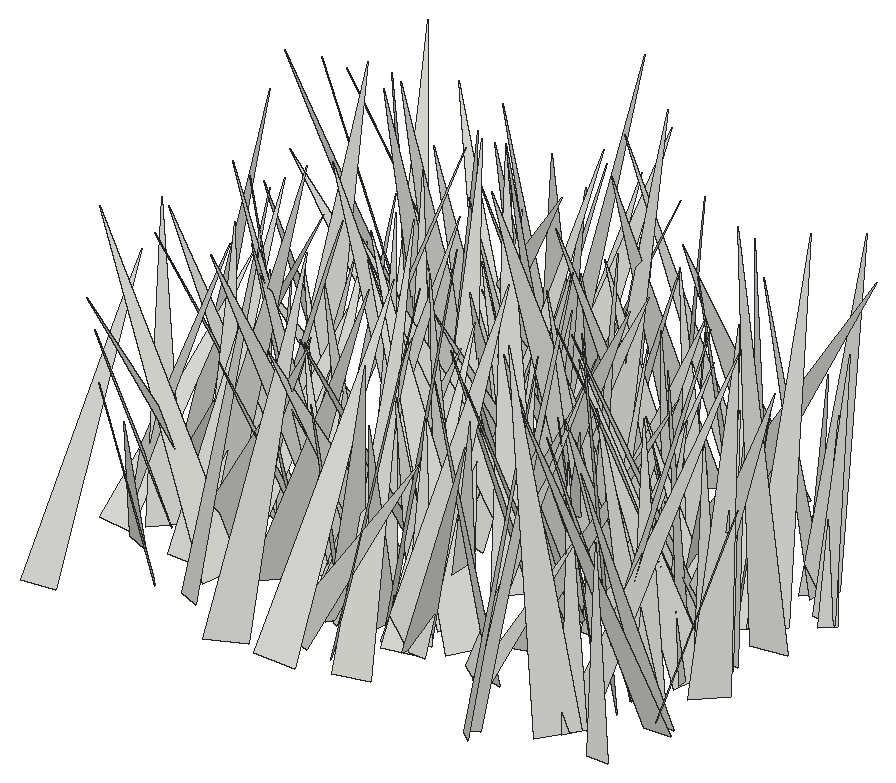
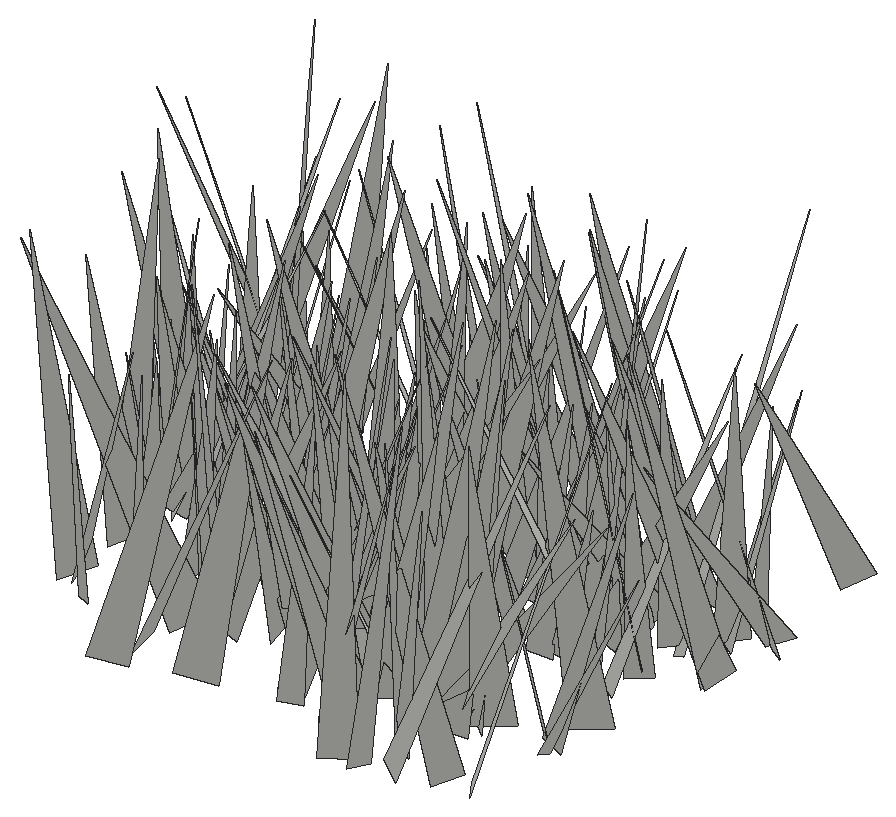
# SketchUp Ruby script. Lengths in inches.
U = 1.inch
M = Sketchup.active_model
def pt(a) = Geom::Point3d.new(a.map { |v| v * U })
def face(e, loops, mat)
  f = e.add_face(loops[0].map { |a| pt(a) })
  loops[1..].each { |l| e.add_face(l.map { |a| pt(a) }).erase! }
  f.material = f.back_material = mat if mat
  f
end
# faces: each face lists its corners as indices into pts; further lists are holes
def faces(e, pts, list, mat = nil) = list.each { |f| face(e, (f[0].is_a?(Array) ? f : [f]).map { |l| l.map { |i| pts[i] } }, mat) }
# xy, xz, yz: faces in a plane at the given z, y or x. An outline is a flat list of corners, or four numbers for a rectangle; further outlines are holes
def ring(l) = l.size == 4 ? [[l[0], l[1]], [l[2], l[1]], [l[2], l[3]], [l[0], l[3]]] : l.each_slice(2).to_a
def flat(e, list, mat, &to3) = list.each { |f| face(e, (f[0].is_a?(Array) ? f : [f]).map { |l| ring(l).map { |u, v| to3.(u, v) } }, mat) }
def xy(e, z, list, mat = nil) = flat(e, list, mat) { |x, y| [x, y, z] }
def xz(e, y, list, mat = nil) = flat(e, list, mat) { |x, z| [x, y, z] }
def yz(e, x, list, mat = nil) = flat(e, list, mat) { |y, z| [x, y, z] }
def lines(e, pts, list) = list.each { |a, b| e.add_line(pt(pts[a]), pt(pts[b])) }
# prism: a flat outline (further loops are holes) pulled along v
def prism(e, loops, v, mat = nil)
  f = face(e, loops, mat); d = Geom::Vector3d.new(v.map { |x| x * U })
  f.pushpull(f.normal.samedirection?(d) ? d.length : -d.length)
end
def box(e, o, s, mat = nil) = prism(e, [[o, [o[0] + s[0], o[1], o[2]], [o[0] + s[0], o[1] + s[1], o[2]], [o[0], o[1] + s[1], o[2]]]], [0, 0, s[2]], mat)
def at(x, y, z, deg = 0) = Geom::Transformation.translation(pt([x, y, z])) * Geom::Transformation.rotation(ORIGIN, Z_AXIS, deg.degrees)
def axes(o, x, y, z) = Geom::Transformation.new([*x, 0, *y, 0, *z, 0, *pt(o).to_a, 1])
def part(name) = M.definitions.add(name)
# library, detail: a bought-in or finely detailed component or shape, given as its bounding box
def library(name, o, s) = part(name).tap { |d| box(d.entities, o, s) }
def detail(e, o, s) = box(e.add_group.entities, o, s)
def put(e, d, t, mat = nil) = e.add_instance(d, t).tap { |i| i.material = mat if mat }
def group(e, t, mat = nil) = e.add_group.tap { |g| g.transformation = t; g.material = mat if mat }.entities
root = M.entities
c1 = part("fur_instance\#9")
p = [[0.8125,0,1.79],[0.67,-0.02,1.48],[0,-0.11,0],[0,0.11,0]]
faces(c1.entities,p,[[0,1,2,3]])
put(root,c1,axes([138.79,216.625,-27.1],[-2.84095,-2.72325,0.75235],[-2.80656,2.8428,-0.30791],[0.32453,0.74533,3.9233]))
put(root,c1,axes([145.17,216.32,-27.1],[2.54302,-4.52945,1.06711],[-4.23804,-1.75205,2.66287],[1.92189,2.12978,4.46004]))
put(root,c1,axes([158.66,216.3125,-27.1],[-0.06677,3.94377,1.582],[4.24655,0.00562,0.16522],[-0.15123,-1.5834,3.94087]))
put(root,c1,axes([143.4,214.84,-27.1],[5.43285,-3.6045,3.64876],[-4.74936,-5.54221,1.59663],[-1.93634,3.48041,6.32132]))
put(root,c1,axes([156.51,216.85,-27.1],[-5.45216,4.70878,2.71596],[5.23215,5.58914,0.81316],[1.47433,-2.42158,7.15803]))
put(root,c1,axes([136.69,218.34,-27.1],[-0.43336,-3.79274,0.22877],[-3.61563,0.48241,1.14868],[1.16807,0.08612,3.64049]))
put(root,c1,axes([135.86,213.875,-27.1],[-4.59878,4.14257,0.47856],[3.69105,4.37512,-2.40275],[1.94062,1.49539,5.70408]))
put(root,c1,axes([146.57,216.95,-27.1],[7.04246,3.4796,1.7186],[3.70112,-7.09298,-0.80545],[-1.16744,-1.49647,7.81378]))
put(root,c1,axes([154.09,214.77,-27.1],[4.5947,4.98178,1.41698],[4.55399,-4.78808,2.06705],[-2.46722,0.43974,6.4542]))
put(root,c1,axes([137.43,221.86,-27.1],[-5.00279,-6.48805,0.18943],[-5.66686,4.48249,3.86684],[3.16501,-2.22958,7.22289]))
put(root,c1,axes([145.65,218.68,-27.1],[5.23742,-3.794,0.7561],[-3.79638,-5.28528,-0.22367],[-0.74406,0.26094,6.46336]))
put(root,c1,axes([145.58,214.8,-27.1],[-1.59566,7.05244,0.57454],[6.94745,1.67322,-1.24356],[1.34162,-0.27674,7.12297]))
put(root,c1,axes([159.07,219.14,-27.1],[-1.75901,-6.72397,0.92553],[-6.70142,1.56883,-1.33876],[-1.07676,1.22044,6.82009]))
put(root,c1,axes([148.83,218.63,-27.1],[5.31861,-1.95589,0.12332],[-1.94358,-5.30997,-0.39374],[-0.25139,-0.32717,5.65315]))
put(root,c1,axes([146.96,219.07,-27.1],[4.83805,-1.95602,0.87332],[-1.75837,-4.85831,-1.14034],[-1.22345,-0.75248,5.09238]))
put(root,c1,axes([152.3,217.64,-27.1],[2.38056,3.51502,0.37387],[3.33138,-2.08023,-1.65431],[1.18197,-1.21634,3.90969]))
put(root,c1,axes([138.8,219.61,-27.1],[2.77166,-6.45652,0.14972],[-5.9267,-2.47813,2.8503],[2.56578,1.25036,6.42219]))
put(root,c1,axes([156.83,217.34,-27.1],[-4.5869,1.43943,1.05541],[1.33614,4.69877,-0.60151],[1.18347,0.27406,4.76967]))
put(root,c1,axes([144.97,219.27,-27.1],[3.60771,1.96245,2.32029],[2.67745,-3.75626,-0.98607],[-1.43745,-2.07119,3.98679]))
put(root,c1,axes([158.9,219.59,-27.1],[-0.82643,-5.48525,0.94931],[-5.54864,0.73423,-0.58792],[-0.44918,1.02229,5.51591]))
put(root,c1,axes([140.375,218.38,-27.1],[-6.66331,2.16551,0.21128],[2.17487,6.60915,0.85019],[-0.06344,-0.87375,6.95459]))
put(root,c1,axes([156.39,220.07,-27.1],[-5.2101,-5.93708,2.74108],[-5.84341,5.80017,1.45611],[2.93548,1.00834,7.76362]))
put(root,c1,axes([136.41,220.42,-27.1],[-3.04266,-3.74721,0.50143],[-3.60797,3.07034,1.05183],[1.12942,-0.28668,4.71094]))
put(root,c1,axes([142.25,221.5,-27.1],[-3.9218,-4.42687,0.35438],[-4.07666,3.77609,2.05553],[1.7617,-1.11678,5.54549]))
put(root,c1,axes([148.41,215.53,-27.1],[0.0768,8.17284,0.16546],[8.06568,-0.10268,1.32775],[-1.3295,-0.15078,8.06464]))
put(root,c1,axes([141.87,219.17,-27.1],[6.48225,-3.39085,0.68777],[-3.4557,-6.41712,0.9323],[-0.17042,1.14593,7.25591]))
put(root,c1,axes([152.53,218.3,-27.1],[-3.42492,-4.02626,1.68032],[-4.34426,2.9504,-1.78518],[-0.40205,2.41841,4.97534]))
put(root,c1,axes([148.8,218.72,-27.1],[-2.37433,3.47563,1.70417],[3.72029,2.6012,-0.12184],[1.06942,-1.33243,4.20745]))
put(root,c1,axes([140.53,216.38,-27.1],[3.83849,6.3713,1.10198],[6.13828,-3.99344,1.70758],[-2.03209,-0.02789,7.23959]))
put(root,c1,axes([144.49,219.02,-27.1],[1.01992,4.1189,1.46608],[4.23417,-0.55549,-1.38501],[1.0893,-1.69737,4.0109]))
put(root,c1,axes([144.74,222.35,-27.1],[-6.04066,-0.63869,2.51357],[0.73038,5.69455,3.20222],[2.48847,-3.22176,5.16172]))
put(root,c1,axes([156.6,220.88,-27.1],[-4.48519,-3.52054,0.94744],[-3.42145,4.58335,0.83384],[1.25916,-0.08621,5.64055]))
put(root,c1,axes([148.57,218.1875,-27.1],[-1.59502,6.99566,2.35908],[7.02793,2.17795,-1.70682],[2.26111,-1.83463,6.96922]))
put(root,c1,axes([146.97,219.4,-27.1],[7.03431,3.48518,2.0857],[3.73576,-7.18871,-0.58711],[-1.59396,-1.46769,7.82836]))
put(root,c1,axes([148.51,221.25,-27.1],[-2.23247,-5.83337,0.18602],[-5.6892,2.13065,-1.46288],[-1.30221,0.692,6.07224]))
put(root,c1,axes([154.09,215.2,-27.1],[4.35175,7.0169,0.44581],[6.16578,-4.0605,3.72408],[-3.37917,1.6275,7.36925]))
put(root,c1,axes([149.11,220.74,-27.1],[4.27597,-2.96302,0.67606],[-2.94629,-4.32773,-0.33261],[-0.74558,0.10858,5.19161]))
put(root,c1,axes([142.72,220.2,-27.1],[-2.07432,-2.92088,0.84042],[-3.01146,2.11274,-0.09003],[0.41107,0.73854,3.58137]))
put(root,c1,axes([147.82,220.33,-27.1],[-3.6167,2.28369,2.19841],[2.80718,3.85669,0.61192],[1.47241,-1.74341,4.23336]))
put(root,c1,axes([144.92,220.76,-27.1],[1.50784,-3.41822,0.5063],[-3.4457,-1.52893,-0.06057],[-0.26023,0.4385,3.73552]))
put(root,c1,axes([143.4,222.04,-27.1],[1.95168,-6.84621,1.26966],[-6.52036,-2.2596,-2.16121],[-2.44285,0.56154,6.78298]))
put(root,c1,axes([144.15,220.08,-27.1],[4.85202,-3.37562,1.03104],[-3.52041,-4.75453,1.00059],[-0.25408,1.41409,5.82544]))
put(root,c1,axes([156.39,218.14,-27.1],[3.64323,6.95762,0.66244],[6.95502,-3.53547,-1.11744],[0.68929,-1.10109,7.77386]))
put(root,c1,axes([158.26,220.34,-27.1],[4.88732,1.92922,0.49219],[1.99044,-4.76555,-1.08522],[-0.04774,-1.19066,5.14102]))
put(root,c1,axes([134.9,219.64,-27.1],[4.20289,4.66758,0.96744],[4.74909,-3.98911,-1.38552],[0.41036,-1.63927,6.12625]))
put(root,c1,axes([150.39,219.59,-27.1],[-4.97351,5.86998,1.15657],[5.9442,4.67754,1.82131],[-0.6788,-2.04794,7.47498]))
put(root,c1,axes([153.36,221.65,-27.1],[-2.96525,-5.05492,0.58848],[-5.08807,2.93137,-0.45808],[-0.10025,0.73898,5.84252]))
put(root,c1,axes([144.8,218.58,-27.1],[3.51205,7.24819,1.1392],[7.33442,-3.43356,-0.76524],[0.20101,-1.35755,8.01781]))
put(root,c1,axes([156.36,218.76,-27.1],[5.62974,5.25868,1.12192],[5.27805,-5.71471,0.30107],[-1.02693,-0.54292,7.69786]))
put(root,c1,axes([144.77,219.97,-27.1],[-7.94923,-1.56442,0.5472],[-1.62855,7.87073,-1.15603],[0.30767,1.24144,8.0188]))
put(root,c1,axes([157.41,220.55,-27.1],[0.3865,-5.10308,2.42648],[-5.49086,-0.91339,-1.04632],[-1.33405,2.28099,5.00959]))
put(root,c1,axes([151.42,218.34,-27.1],[3.77289,4.9439,0.17652],[4.9129,-3.7705,0.5956],[-0.58026,0.22179,6.19049]))
put(root,c1,axes([139.36,220.99,-27.1],[3.2608,1.42212,0.87051],[1.60342,-3.19897,-0.78016],[-0.45742,-1.07574,3.47082]))
put(root,c1,axes([136.67,219.89,-27.1],[-4.60516,3.74944,1.60687],[3.84875,4.79672,-0.16237],[1.35183,-0.88372,5.93628]))
put(root,c1,axes([140.39,219.43,-27.1],[4.26964,0.47793,1.18834],[0.14194,-4.28676,1.21405],[-1.27296,1.12502,4.1212]))
put(root,c1,axes([138.6,219.76,-27.1],[7.3545,-2.24014,2.18394],[-2.66673,-7.40612,1.38362],[-1.63595,2.00191,7.56257]))
put(root,c1,axes([157.34,220.75,-27.1],[2.70237,-4.42657,2.31196],[-4.83243,-2.98105,-0.05917],[-1.25989,1.93941,5.18593]))
put(root,c1,axes([148.54,218,-27.1],[-4.13598,4.27474,0.09369],[4.07434,3.97972,-1.71759],[1.29691,1.13001,5.6947]))
put(root,c1,axes([148.81,220.54,-27.1],[-1.16984,-6.03511,2.92768],[-6.70455,0.96018,-0.69968],[-0.2073,3.00298,6.1075]))
put(root,c1,axes([144.25,220.6,-27.1],[2.31719,-2.3997,1.71249],[-2.74416,-2.55172,0.13746],[-1.07739,1.33819,3.33302]))
put(root,c1,axes([151.54,223.72,-27.1],[6.17469,-3.94346,0.96595],[-3.5616,-6.10514,-2.15707],[-1.94909,-1.33681,7.00177]))
put(root,c1,axes([149.03,220.72,-27.1],[-5.22041,4.31379,0.87725],[4.39805,5.05275,1.32586],[-0.18846,-1.57859,6.64105]))
put(root,c1,axes([143.22,220.8,-27.1],[-3.14224,2.77876,1.0294],[2.91205,3.17344,0.32264],[0.54877,-0.92877,4.18224]))
put(root,c1,axes([138.76,218.4,-27.1],[0.11708,7.08162,0.20269],[7.08451,-0.11681,-0.01106],[0.00771,-0.20285,7.08258]))
put(root,c1,axes([154.96,220.86,-27.1],[-3.71707,-2.68533,1.32909],[-2.9797,3.53518,-1.19076],[0.31439,1.75658,4.42828]))
put(root,c1,axes([146.03,220.1,-27.1],[0.42916,7.00561,1.64499],[7.11073,-0.66598,0.98114],[-1.10544,-1.56418,6.94983]))
put(root,c1,axes([157.76,222.74,-27.1],[-5.95975,2.47486,1.75961],[2.91321,5.75356,1.77469],[0.85695,-2.34763,6.20435]))
put(root,c1,axes([156.88,224.47,-27.1],[-5.73536,-5.62008,0.65862],[-5.46135,5.74328,1.44982],[1.48081,-0.58562,7.89796]))
put(root,c1,axes([135.26,218.88,-27.1],[-2.44099,4.81015,0.04297],[4.37742,2.2412,-2.21652],[1.99437,0.96814,4.91762]))
put(root,c1,axes([151.91,223.63,-27.1],[-0.76321,-4.71965,0.1503],[-4.6984,0.77422,0.45372],[0.47201,0.07524,4.75939]))
put(root,c1,axes([140.65,223.77,-27.1],[-0.18064,-6.52008,0.8881],[-6.57997,0.17015,-0.08916],[-0.06535,0.89016,6.52198]))
put(root,c1,axes([137.96,221.34,-27.1],[3.60386,-3.42869,2.87422],[-4.08632,-4.02533,0.32181],[-1.82182,2.24626,4.96388]))
put(root,c1,axes([151.09,224.28,-27.1],[-0.50575,-5.47671,0.42869],[-5.44927,0.55465,0.65709],[0.69543,0.36321,5.46062]))
put(root,c1,axes([138.57,225.09,-27.1],[-4.91582,-6.36103,2.07601],[-5.8042,5.33544,2.60426],[3.32923,-0.09063,7.60565]))
put(root,c1,axes([137.95,223.26,-27.1],[5.79589,4.16761,1.50359],[4.42839,-5.37215,-2.17978],[0.13803,-2.64446,6.79779]))
put(root,c1,axes([137.8125,225.34,-27.1],[-3.98509,-5.15803,0.00595],[-5.07141,3.91953,1.18509],[0.94137,-0.71992,6.40951]))
put(root,c1,axes([151.54,220.64,-27.1],[5.52796,-0.81869,0.7417],[-1.07099,-4.89962,2.57397],[-0.27083,2.66498,4.96017]))
put(root,c1,axes([140.28,222.67,-27.1],[-1.81659,5.58818,1.87966],[5.39696,0.78429,2.88421],[-2.37355,-2.49359,5.11948]))
put(root,c1,axes([158.39,222.79,-27.1],[-3.98978,2.11987,2.03955],[2.3526,4.36264,0.06771],[1.76604,-1.02247,4.51748]))
put(root,c1,axes([139.4,222.57,-27.1],[1.95895,3.98258,1.69888],[4.26762,-2.09086,-0.01944],[-0.73116,-1.53362,4.43825]))
put(root,c1,axes([135.21,222.33,-27.1],[6.85637,-0.90607,0.05149],[-0.90407,-6.7849,0.99057],[0.07926,0.98874,6.84468]))
put(root,c1,axes([149.9,223.8,-27.1],[-2.91722,-4.26379,0.81225],[-4.33997,2.88016,-0.46811],[0.06569,0.93518,5.14499]))
put(root,c1,axes([158.99,222.14,-27.1],[5.64429,-3.09602,3.33103],[-3.78051,-6.14532,0.69416],[-2.52761,2.27789,6.40012]))
put(root,c1,axes([158.16,223.8125,-27.1],[2.54214,-2.62214,0.84113],[-2.70032,-2.59808,0.06187],[-0.53981,0.64801,3.65161]))
put(root,c1,axes([139.62,220.21,-27.1],[-3.68567,4.23937,0.30212],[3.60627,3.33103,-2.74713],[2.24908,1.60613,4.89997]))
put(root,c1,axes([157.61,224.69,-27.1],[-5.40162,-4.18627,0.13743],[-4.18531,5.38577,-0.4449],[-0.16419,0.43574,6.81941]))
put(root,c1,axes([152.88,225.24,-27.1],[2.25117,-4.50739,0.41367],[-4.42833,-2.28883,-0.84056],[-0.93676,-0.01195,4.96767]))
put(root,c1,axes([137.53,223.91,-27.1],[-2.45808,3.26284,2.53045],[3.74921,2.99751,-0.22312],[1.72995,-1.86016,4.07903]))
put(root,c1,axes([157.625,222.51,-27.1],[-5.30333,-1.20318,1.41609],[-1.56427,5.2022,-1.4382],[1.00301,1.75149,5.24448]))
put(root,c1,axes([141.08,221.875,-27.1],[-2.87102,4.68172,0.40163],[4.57171,2.89185,-1.02921],[1.08596,0.20316,5.39463]))
put(root,c1,axes([142.53,224.25,-27.1],[1.52627,-4.48364,1.33128],[-4.39877,-0.90019,2.01128],[1.58937,1.81423,4.28804]))
put(root,c1,axes([156.03,224.47,-27.1],[3.29636,-5.4576,1.30622],[-5.51274,-2.86598,1.93739],[1.04942,2.08768,6.07437]))
put(root,c1,axes([141.25,224.82,-27.1],[0.46643,-4.66615,1.44002],[-4.86096,-0.58186,-0.31092],[-0.46655,1.39737,4.67909]))
put(root,c1,axes([135.65,222.11,-27.1],[-6.79191,0.51616,3.38033],[-0.49773,7.28774,-2.11287],[3.3831,2.10844,6.47551]))
put(root,c1,axes([144.375,225.44,-27.1],[4.0303,-5.81988,3.12764],[-5.66664,-4.92868,-1.86917],[-3.39741,1.31665,6.82792]))
put(root,c1,axes([157.97,223.84,-27.1],[-2.87037,3.7349,1.34525],[3.80013,3.06525,-0.40189],[1.14815,-0.80807,4.69329]))
put(root,c1,axes([149.66,226.02,-27.1],[4.03439,-1.67825,0.01541],[-1.64329,-3.95818,-0.85174],[-0.3411,-0.78061,4.28572]))
put(root,c1,axes([154.6,226.28,-27.1],[4.66467,-0.77947,0.02704],[-0.7406,-4.47818,-1.32848],[-0.24456,-1.30606,4.53893]))
put(root,c1,axes([149.18,223.625,-27.1],[-6.71454,4.39928,1.56364],[4.39375,6.8803,-0.4901],[1.57912,-0.43767,8.0124]))
put(root,c1,axes([154.5625,224.64,-27.1],[0.69151,3.97199,1.28395],[4.17346,-0.6309,-0.296],[0.08642,-1.31479,4.02085]))
put(root,c1,axes([157.38,224.82,-27.1],[-1.85647,3.95367,0.8299],[3.82368,1.42492,1.76516],[-1.30372,-1.4508,3.99527]))
put(root,c1,axes([152.96,223.03,-27.1],[2.80201,6.02167,1.40008],[5.6342,-3.12002,2.14317],[-2.54489,-0.27744,6.28638]))
put(root,c1,axes([147.13,226.45,-27.1],[3.33833,-6.51025,0.54896],[-6.14625,-2.92038,2.74304],[2.21549,1.70799,6.78259]))
put(root,c1,axes([152.72,224.22,-27.1],[2.02103,5.13059,0.73898],[5.12624,-1.86067,-1.10143],[0.76856,-1.08099,5.40318]))
put(root,c1,axes([147.71,226.36,-27.1],[-4.43221,4.72995,1.58971],[4.78005,3.41433,3.16821],[-1.43205,-3.24253,5.65503]))
put(root,c1,axes([158.14,224.45,-27.1],[1.43677,3.63281,1.03111],[3.57622,-1.66329,0.8769],[-1.21291,-0.60083,3.80693]))
put(root,c1,axes([151.29,225.66,-27.1],[-5.71627,0.02456,1.51927],[0.09668,5.9079,0.26822],[1.51639,-0.28405,5.71003]))
put(root,c1,axes([140.52,224.46,-27.1],[-1.14245,4.14217,0.46464],[4.01441,0.96381,1.27839],[-1.12161,-0.76952,4.10226]))
put(root,c1,axes([140.23,223.15,-27.1],[5.64336,5.1887,0.30355],[5.15395,-5.64438,0.66329],[-0.67191,0.28398,7.63742]))
put(root,c1,axes([148.5625,226.45,-27.1],[-1.63509,-3.83691,0.93062],[-3.94815,1.58786,-0.39017],[-0.00453,1.00909,4.15248]))
put(root,c1,axes([145.66,227.8,-27.1],[-0.82646,-4.24361,0.01629],[-4.06802,0.79698,1.2278],[1.20816,-0.21938,4.14533]))
put(root,c1,axes([148.79,224.56,-27.1],[-4.40287,4.25609,0.42122],[4.26988,4.40886,0.08361],[0.24458,-0.35298,6.12311]))
put(root,c1,axes([149.28,228.42,-27.1],[5.28612,-6.00356,2.19792],[-5.60526,-5.72373,-2.15328],[-3.07484,0.113,7.70384]))
put(root,c1,axes([146.87,228.92,-27.1],[-4.92711,-3.11526,0.5387],[-2.69685,4.66208,2.29422],[1.64986,-1.68274,5.3589]))
put(root,c1,axes([148.49,224.375,-27.1],[-4.43133,1.84787,0.51045],[1.62369,4.30117,-1.47494],[1.01922,1.18203,4.56901]))
put(root,c1,axes([154.4375,226.51,-27.1],[-2.57629,-2.49445,0.93197],[-2.62206,2.60252,-0.28257],[0.46438,0.85602,3.57488]))
put(root,c1,axes([145.41,224.82,-27.1],[-2.63415,6.93544,1.64719],[7.09873,2.71215,-0.06728],[0.64926,-1.51533,7.41852]))
put(root,c1,axes([154.34,225.92,-27.1],[-5.10853,0.04095,1.59169],[-0.11644,5.32521,-0.51071],[1.58796,0.52222,5.08311]))
put(root,c1,axes([158.49,226.05,-27.1],[-0.94907,-6.99906,3.73248],[-7.88487,0.42284,-1.21201],[-0.8643,3.82797,6.95835]))
put(root,c1,axes([147.15,226.8,-27.1],[-4.76846,2.17787,1.48985],[2.383,4.8757,0.4998],[1.13316,-1.08876,5.21838]))
put(root,c1,axes([149.72,225.72,-27.1],[-6.70794,-1.60484,0.19836],[-1.59675,6.44001,-1.8942],[-0.25542,1.88735,6.63204]))
put(root,c1,axes([137.375,226.74,-27.1],[1.77196,3.84512,1.4323],[4.08534,-1.50774,-1.0065],[0.38272,-1.70823,4.11239]))
put(root,c1,axes([146.46,227.3,-27.1],[0.92533,-3.44435,1.34936],[-3.58141,-1.18238,-0.56215],[-0.92618,1.13092,3.52189]))
put(root,c1,axes([143.45,225.4375,-27.1],[-0.40472,6.25604,0.83945],[6.18781,0.22712,1.29072],[-1.24649,-0.90382,6.13481]))
put(root,c1,axes([145.23,226.2,-27.1],[3.77133,0.16267,0.95437],[-0.10228,-3.74984,1.04331],[-0.96272,1.03561,3.6278]))
put(root,c1,axes([144.08,229.67,-27.1],[4.85347,-3.26157,0.26621],[-3.0891,-4.72355,-1.55255],[-1.07988,-1.1468,5.6377]))
put(root,c1,axes([151.6,225.61,-27.1],[1.45734,4.18221,0.34787],[4.02467,-1.49715,1.13854],[-1.18907,0.05834,4.28]))
put(root,c1,axes([146.98,227.25,-27.1],[4.06657,-2.17936,1.39694],[-2.40276,-4.14574,0.52683],[-0.9632,1.14071,4.58356]))
put(root,c1,axes([155.69,228.37,-27.1],[-5.52938,-3.456,2.07939],[-3.45701,5.87854,0.57763],[2.07771,0.58365,6.49494]))
put(root,c1,axes([156.48,226.76,-27.1],[3.3556,2.16226,1.21696],[2.08771,-3.56664,0.58052],[-1.34083,-0.14202,3.94948]))
put(root,c1,axes([146.54,228.1,-27.1],[2.73482,-5.11249,1.4467],[-5.08402,-2.04521,2.38319],[1.54377,2.32148,5.28557]))
put(root,c1,axes([156.95,226.78,-27.1],[-1.86757,4.60063,0.33127],[4.58089,1.80817,0.71369],[-0.53944,-0.57279,4.91369]))
put(root,c1,axes([145.72,225.44,-27.1],[2.14003,7.20036,0.0672],[7.19519,-2.14104,0.27303],[-0.28086,0.01341,7.50668]))
put(root,c1,axes([136.58,227.76,-27.1],[-2.68799,6.56885,2.98447],[6.8694,3.30396,-1.08507],[2.20641,-2.2839,7.01411]))
put(root,c1,axes([149.5625,228.29,-27.1],[-0.77235,4.89048,2.70767],[4.92537,1.88806,-2.00519],[2.64368,-2.08884,4.52687]))
put(root,c1,axes([136.89,229.58,-27.1],[-1.73362,-4.79917,0.85478],[-4.86621,1.65027,-0.60395],[-0.28757,1.00633,5.06683]))
put(root,c1,axes([141.82,229.5,-27.1],[7.52805,-0.18805,1.99939],[0.07054,-7.72753,-0.99239],[-2.00698,-0.97696,7.46472]))
put(root,c1,axes([136.75,230.1875,-27.1],[-3.56897,-0.50146,0.42511],[-0.28446,3.29362,1.49696],[0.59267,-1.43888,3.27843]))
put(root,c1,axes([143.22,230.29,-27.1],[-6.0404,2.2493,3.21945],[3.13358,6.3206,1.46334],[2.36747,-2.62704,6.2773]))
put(root,c1,axes([154.05,227.9375,-27.1],[-5.59826,1.4556,0.99849],[1.35798,5.67289,-0.65612],[1.12768,0.39476,5.74707]))
put(root,c1,axes([147.16,229.89,-27.1],[-0.83843,-4.56243,0.7415],[-4.45874,0.59959,-1.35228],[-1.2187,0.94513,4.43735]))
put(root,c1,axes([144.71,227.39,-27.1],[-3.134,4.47853,0.59876],[4.43295,3.18866,-0.64743],[0.8745,-0.1137,5.42771]))
put(root,c1,axes([147.93,228.45,-27.1],[1.92341,3.31368,0.82854],[3.39872,-1.95136,-0.08567],[-0.34002,-0.7604,3.83049]))
put(root,c1,axes([157.47,227.27,-27.1],[-5.92088,3.75972,1.43779],[3.50525,6.07307,-1.44586],[1.97886,0.49178,6.86307]))
put(root,c1,axes([150.875,230.3,-27.1],[-1.01411,-6.0227,1.51425],[-5.97973,0.53295,-1.88497],[-1.67593,1.7428,5.80932]))
put(root,c1,axes([149.61,227.76,-27.1],[1.82525,7.99707,1.79582],[8.16577,-1.93273,0.30716],[-0.70587,-1.67961,8.19697]))
put(root,c1,axes([140.36,231.04,-27.1],[1.08245,-7.41016,1.80762],[-7.58562,-1.23679,-0.52762],[-0.7977,1.70574,7.47019]))
put(root,c1,axes([158.65,228.88,-27.1],[0.70725,4.81258,1.31899],[4.97344,-0.78845,0.21001],[-0.40688,-1.27212,4.85974]))
put(root,c1,axes([159.04,228.6,-27.1],[-3.45785,1.40655,0.59459],[1.25916,3.45892,-0.85969],[0.86397,0.58836,3.63264]))
put(root,c1,axes([141.34,231.02,-27.1],[1.42395,-7.42701,2.10024],[-7.62151,-1.69014,-0.80943],[-1.21824,1.89264,7.51884]))
put(root,c1,axes([150.9375,230.49,-27.1],[4.1746,-2.61988,2.8232],[-2.37692,-5.02847,-1.15163],[-3.03059,0.33503,4.79215]))
put(root,c1,axes([146.28,232.25,-27.1],[3.38656,-3.48151,1.0277],[-2.77448,-3.38882,-2.33752],[-2.3408,-1.02022,4.25743]))
put(root,c1,axes([148.71,228.75,-27.1],[5.15508,0.33774,1.32609],[0.02228,-5.18864,1.23487],[-1.36825,1.188,5.01637]))
put(root,c1,axes([139.91,229.9375,-27.1],[-4.37552,-5.12362,2.64469],[-5.63456,4.50416,-0.59611],[1.22377,2.41912,6.71129]))
put(root,c1,axes([145.33,230.84,-27.1],[-6.26815,-2.22604,2.13273],[-2.17784,6.6177,0.5065],[2.18193,0.21043,6.63238]))
put(root,c1,axes([140.89,230.72,-27.1],[-3.83855,4.56526,0.77541],[4.17711,2.97899,3.13921],[-1.99865,-2.54191,5.07163]))
put(root,c1,axes([137.43,229.23,-27.1],[2.58432,3.47984,0.90101],[3.42396,-2.72089,0.68775],[-1.09434,-0.29537,4.2796]))
put(root,c1,axes([145.52,228.67,-27.1],[6.4283,2.09347,0.22673],[2.03253,-6.35917,1.08941],[-0.55031,0.96716,6.67224]))
put(root,c1,axes([149,228.33,-27.1],[-5.03448,1.97141,0.87824],[1.57247,4.87743,-1.93439],[1.47821,1.52579,5.04882]))
put(root,c1,axes([150.87,230.24,-27.1],[5.91365,2.78735,2.33328],[2.94924,-6.28377,0.03183],[-2.12497,-0.96423,6.53755]))
put(root,c1,axes([145.21,230.45,-27.1],[5.91491,-0.67607,1.90084],[-0.77835,-6.19702,0.21795],[-1.8613,0.44302,5.94943]))
put(root,c1,axes([152.07,230.52,-27.1],[6.07863,-4.42165,0.21276],[-4.21796,-5.67554,2.55792],[1.3435,2.18706,7.06807]))
put(root,c1,axes([157.35,230.16,-27.1],[-5.62081,-1.07857,0.79033],[-1.22962,5.511,-1.22409],[0.52534,1.35906,5.59093]))
put(root,c1,axes([149.22,229.18,-27.1],[-5.01986,0.40192,1.5189],[-0.17545,4.90978,-1.87904],[1.56135,1.84392,4.67223]))
put(root,c1,axes([157.33,230.28,-27.1],[-5.57842,3.33095,2.99608],[3.28064,6.29556,-0.89096],[3.05108,-0.67911,6.43585]))
put(root,c1,axes([145.85,232.86,-27.1],[0.34868,-5.31048,0.36463],[-5.26358,-0.28954,0.81646],[0.79301,0.41316,5.25892]))
put(root,c1,axes([137.14,233.73,-27.1],[-6.21102,-4.85766,0.88936],[-4.64444,6.23147,1.60082],[1.67841,-0.73247,7.72082]))
put(root,c1,axes([149.47,233.55,-27.1],[2.6009,-7.25193,0.96085],[-7.2129,-2.71231,-0.94648],[-1.21974,0.57558,7.64587]))
put(root,c1,axes([149.94,232.45,-27.1],[4.17117,1.8451,1.43695],[2.27213,-3.89306,-1.59669],[-0.55375,-2.07548,4.27243]))
put(root,c1,axes([156,231.63,-27.1],[-1.72893,-3.46771,1.76985],[-3.62718,2.13831,0.64633],[1.41454,1.24466,3.82053]))
put(root,c1,axes([141.12,229.99,-27.1],[-6.11447,-3.98639,0.59028],[-3.68819,5.10346,-3.73879],[-1.62389,3.41906,6.26894]))
put(root,c1,axes([143.76,230.22,-27.1],[-4.22823,5.63878,0.60494],[5.64653,4.11564,1.10357],[-0.52773,-1.14251,6.96102]))
put(root,c1,axes([144.16,233.38,-27.1],[-4.57132,-4.01454,0.83204],[-3.89365,4.6413,1.00178],[1.28384,-0.21818,6.00082]))
put(root,c1,axes([138.18,233.71,-27.1],[1.13503,-7.67663,0.6742],[-6.50823,-0.58999,4.2389],[4.12651,1.18099,6.50005]))
put(root,c1,axes([152.65,234.48,-27.1],[3.73251,-5.71066,0.85994],[-5.41751,-3.81707,-1.83396],[-2.00044,-0.31799,6.57114]))
put(root,c1,axes([139.35,229.7,-27.1],[-4.20767,6.2047,0.57896],[6.20765,4.23458,-0.26697],[0.54635,-0.32858,7.49209]))
put(root,c1,axes([144.33,229.1875,-27.1],[3.4696,4.95294,0.18512],[4.68916,-3.35343,1.83583],[-1.60551,0.90933,5.7619]))
put(root,c1,axes([141.11,232.52,-27.1],[5.21956,1.10973,1.69595],[1.36173,-5.39042,-0.66376],[-1.50115,-1.03121,5.29478]))
put(root,c1,axes([154.13,231.05,-27.1],[-5.50715,-0.70612,1.61288],[-1.08889,5.52799,-1.29784],[1.38358,1.53996,5.39842]))
put(root,c1,axes([140.17,234.45,-27.1],[-4.57477,-6.03245,0.25242],[-6.03633,4.57654,-0.02819],[0.13005,0.21817,7.57088]))
put(root,c1,axes([146.06,228.55,-27.1],[7.29611,1.84526,3.54482],[-0.04664,-7.33917,3.91643],[-3.99607,3.45479,6.4265]))
put(root,c1,axes([152.49,232.75,-27.1],[-7.29173,-1.24054,0.1592],[-1.24954,7.26646,-0.60898],[0.05425,0.6271,7.37139]))
put(root,c1,axes([144.55,231.06,-27.1],[-2.83058,6.09964,1.95872],[5.76034,3.3604,-2.14023],[2.80369,-0.74599,6.37473]))
put(root,c1,axes([142.11,234.89,-27.1],[2.97455,-6.14482,0.55918],[-6.16848,-2.94679,0.43089],[0.14598,0.69067,6.8133]))
put(root,c1,axes([140.75,233.08,-27.1],[1.70203,4.17643,2.24286],[4.55719,-2.09788,0.44817],[-1.30578,-1.87783,4.48761]))
put(root,c1,axes([143.98,232.16,-27.1],[0.03547,5.69131,1.501],[5.73382,0.30561,-1.29426],[1.32938,-1.46999,5.5423]))
put(root,c1,axes([144.48,232.39,-27.1],[-6.24639,-1.28271,0.8155],[-1.43317,6.11916,-1.35263],[0.50635,1.49608,6.23162]))
put(root,c1,axes([141.22,234.86,-27.1],[5.81845,-0.62274,2.18855],[-0.03101,-6.03017,-1.6334],[-2.27522,-1.51035,5.61909]))
